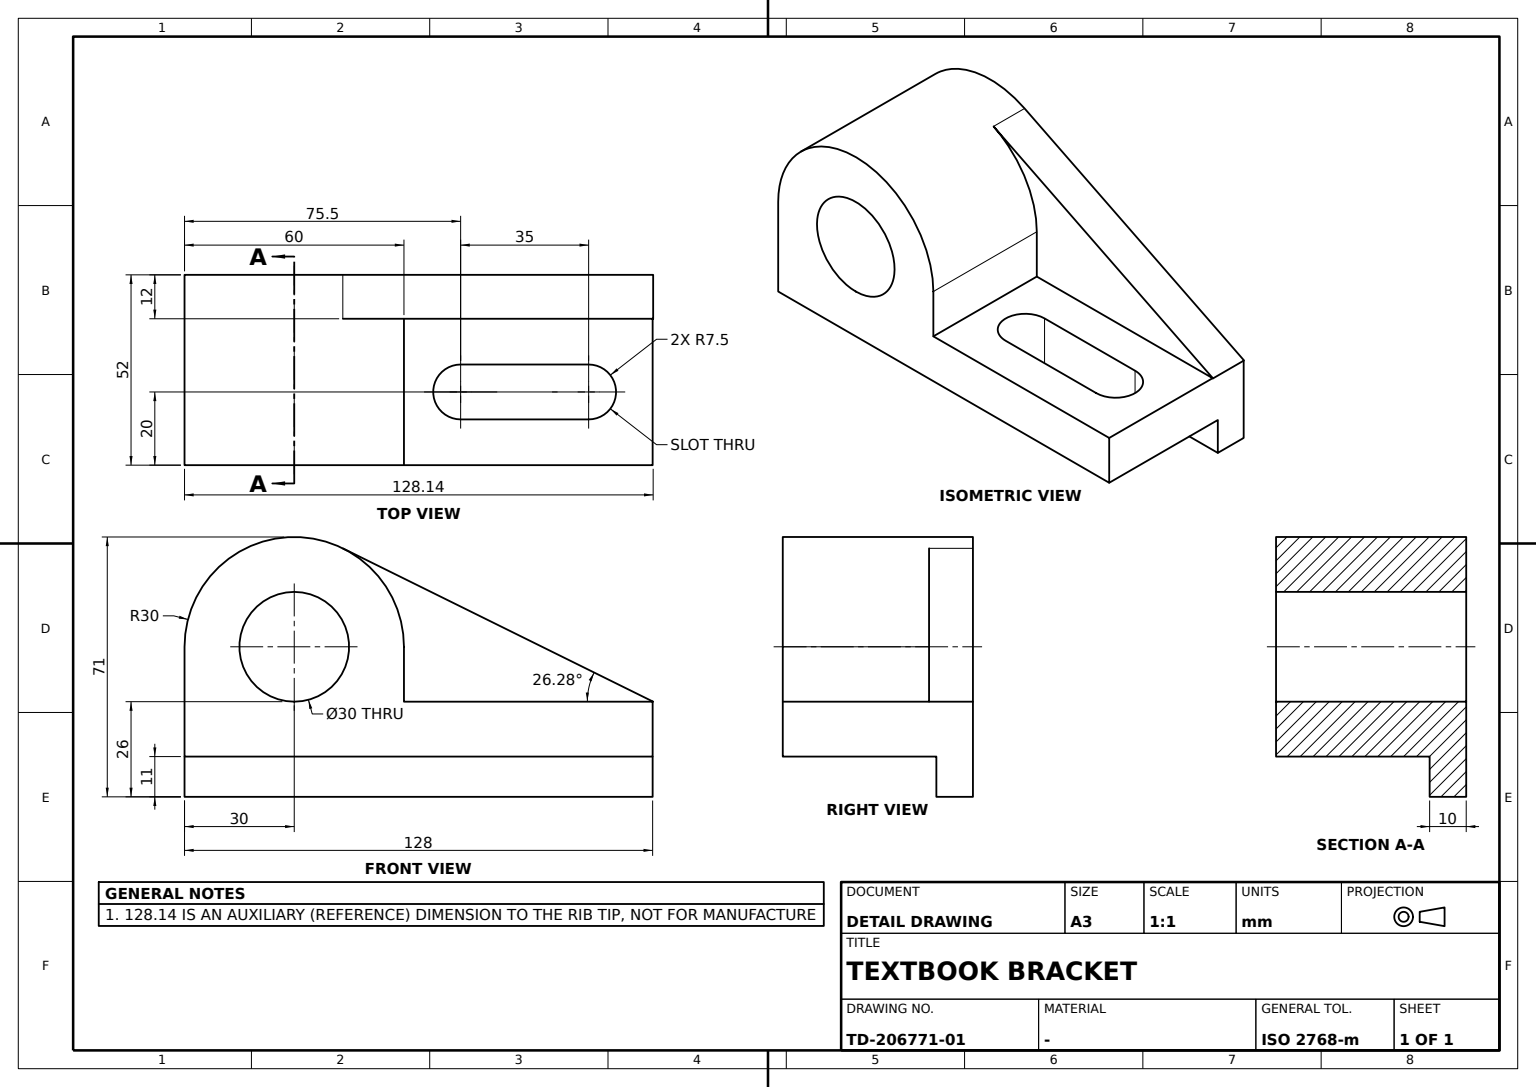
ISO-10303-21;
HEADER;
FILE_DESCRIPTION((''),'2;1');
FILE_NAME('','',(''),(''),'','','');
FILE_SCHEMA(('AUTOMOTIVE_DESIGN'));
ENDSEC;
DATA;
#1=APPLICATION_CONTEXT('');
#2=PRODUCT_CONTEXT('',#1,'mechanical');
#3=PRODUCT('','','',(#2));
#4=PRODUCT_DEFINITION_FORMATION('','',#3);
#5=PRODUCT_DEFINITION_CONTEXT('',#1,'design');
#6=PRODUCT_DEFINITION('','',#4,#5);
#7=PRODUCT_DEFINITION_SHAPE('','',#6);
#8=(LENGTH_UNIT()NAMED_UNIT(*)SI_UNIT(.MILLI.,.METRE.));
#9=(NAMED_UNIT(*)PLANE_ANGLE_UNIT()SI_UNIT($,.RADIAN.));
#10=(NAMED_UNIT(*)SI_UNIT($,.STERADIAN.)SOLID_ANGLE_UNIT());
#11=UNCERTAINTY_MEASURE_WITH_UNIT(LENGTH_MEASURE(0.005),#8,'distance_accuracy_value','');
#12=(GEOMETRIC_REPRESENTATION_CONTEXT(3)GLOBAL_UNCERTAINTY_ASSIGNED_CONTEXT((#11))GLOBAL_UNIT_ASSIGNED_CONTEXT((#8,#9,#10))REPRESENTATION_CONTEXT('',''));
#13=CARTESIAN_POINT('',(26.,-30.,0.));
#14=VERTEX_POINT('',#13);
#15=CARTESIAN_POINT('',(26.,-30.,-30.));
#16=VERTEX_POINT('',#15);
#17=DIRECTION('',(0.,0.,-1.));
#18=VECTOR('',#17,1000.);
#19=LINE('',#13,#18);
#20=EDGE_CURVE('',#14,#16,#19,.T.);
#21=ORIENTED_EDGE('',*,*,#20,.T.);
#22=CARTESIAN_POINT('',(26.,98.,-30.));
#23=VERTEX_POINT('',#22);
#24=CARTESIAN_POINT('',(26.,0.,-30.));
#25=DIRECTION('',(0.,1.,0.));
#26=VECTOR('',#25,1000.);
#27=LINE('',#24,#26);
#28=EDGE_CURVE('',#16,#23,#27,.T.);
#29=ORIENTED_EDGE('',*,*,#28,.T.);
#30=CARTESIAN_POINT('',(26.,98.,-15.));
#31=VERTEX_POINT('',#30);
#32=CARTESIAN_POINT('',(26.,98.,0.));
#33=DIRECTION('',(0.,0.,1.));
#34=VECTOR('',#33,1000.);
#35=LINE('',#32,#34);
#36=EDGE_CURVE('',#23,#31,#35,.T.);
#37=ORIENTED_EDGE('',*,*,#36,.T.);
#38=CARTESIAN_POINT('',(26.,30.,-15.));
#39=VERTEX_POINT('',#38);
#40=CARTESIAN_POINT('',(26.,0.,-15.));
#41=DIRECTION('',(0.,-1.,0.));
#42=VECTOR('',#41,1000.);
#43=LINE('',#40,#42);
#44=EDGE_CURVE('',#31,#39,#43,.T.);
#45=ORIENTED_EDGE('',*,*,#44,.T.);
#46=CARTESIAN_POINT('',(26.,30.,0.));
#47=VERTEX_POINT('',#46);
#48=LINE('',#46,#34);
#49=EDGE_CURVE('',#39,#47,#48,.T.);
#50=ORIENTED_EDGE('',*,*,#49,.T.);
#51=CARTESIAN_POINT('',(26.,0.,0.));
#52=DIRECTION('',(1.,0.,0.));
#53=AXIS2_PLACEMENT_3D('',#51,#52,#17);
#54=CIRCLE('',#53,30.);
#55=EDGE_CURVE('',#47,#14,#54,.T.);
#56=ORIENTED_EDGE('',*,*,#55,.T.);
#57=EDGE_LOOP('',(#21,#29,#37,#45,#50,#56));
#58=FACE_BOUND('',#57,.T.);
#59=VERTEX_POINT('',#40);
#60=CIRCLE('',#53,15.);
#61=EDGE_CURVE('',#59,#59,#60,.T.);
#62=ORIENTED_EDGE('',*,*,#61,.F.);
#63=EDGE_LOOP('',(#62));
#64=FACE_BOUND('',#63,.T.);
#65=AXIS2_PLACEMENT_3D('',#51,#52,#25);
#66=PLANE('',#65);
#67=ADVANCED_FACE('',(#58,#64),#66,.T.);
#68=CARTESIAN_POINT('',(-16.,98.,-41.));
#69=VERTEX_POINT('',#68);
#70=CARTESIAN_POINT('',(-16.,-30.,-41.));
#71=VERTEX_POINT('',#70);
#72=LINE('',#68,#42);
#73=EDGE_CURVE('',#69,#71,#72,.T.);
#74=ORIENTED_EDGE('',*,*,#73,.T.);
#75=CARTESIAN_POINT('',(-26.,-30.,-41.));
#76=VERTEX_POINT('',#75);
#77=CARTESIAN_POINT('',(0.,-30.,-41.));
#78=VECTOR('',#52,1000.);
#79=LINE('',#77,#78);
#80=EDGE_CURVE('',#76,#71,#79,.T.);
#81=ORIENTED_EDGE('',*,*,#80,.F.);
#82=CARTESIAN_POINT('',(-26.,98.,-41.));
#83=VERTEX_POINT('',#82);
#84=LINE('',#82,#42);
#85=EDGE_CURVE('',#83,#76,#84,.T.);
#86=ORIENTED_EDGE('',*,*,#85,.F.);
#87=LINE('',#82,#78);
#88=EDGE_CURVE('',#83,#69,#87,.T.);
#89=ORIENTED_EDGE('',*,*,#88,.T.);
#90=EDGE_LOOP('',(#74,#81,#86,#89));
#91=FACE_BOUND('',#90,.T.);
#92=AXIS2_PLACEMENT_3D('',#82,#17,#52);
#93=PLANE('',#92);
#94=ADVANCED_FACE('',(#91),#93,.T.);
#95=CARTESIAN_POINT('',(-14.,30.,0.));
#96=VERTEX_POINT('',#95);
#97=CARTESIAN_POINT('',(-14.,13.281713,26.899742));
#98=VERTEX_POINT('',#97);
#99=CARTESIAN_POINT('',(-14.,0.,0.));
#100=AXIS2_PLACEMENT_3D('',#99,#52,#17);
#101=CIRCLE('',#100,30.);
#102=EDGE_CURVE('',#96,#98,#101,.T.);
#103=ORIENTED_EDGE('',*,*,#102,.T.);
#104=CARTESIAN_POINT('',(-26.,13.281713,26.899742));
#105=VERTEX_POINT('',#104);
#106=CARTESIAN_POINT('',(0.,13.281713,26.899742));
#107=LINE('',#106,#78);
#108=EDGE_CURVE('',#105,#98,#107,.T.);
#109=ORIENTED_EDGE('',*,*,#108,.F.);
#110=CARTESIAN_POINT('',(-26.,-30.,0.));
#111=VERTEX_POINT('',#110);
#112=CARTESIAN_POINT('',(-26.,0.,0.));
#113=AXIS2_PLACEMENT_3D('',#112,#52,#17);
#114=CIRCLE('',#113,30.);
#115=EDGE_CURVE('',#105,#111,#114,.T.);
#116=ORIENTED_EDGE('',*,*,#115,.T.);
#117=CARTESIAN_POINT('',(0.,-30.,0.));
#118=LINE('',#117,#78);
#119=EDGE_CURVE('',#111,#14,#118,.T.);
#120=ORIENTED_EDGE('',*,*,#119,.T.);
#121=ORIENTED_EDGE('',*,*,#55,.F.);
#122=CARTESIAN_POINT('',(0.,30.,0.));
#123=LINE('',#122,#78);
#124=EDGE_CURVE('',#96,#47,#123,.T.);
#125=ORIENTED_EDGE('',*,*,#124,.F.);
#126=EDGE_LOOP('',(#103,#109,#116,#120,#121,#125));
#127=FACE_BOUND('',#126,.T.);
#128=CARTESIAN_POINT('',(0.,0.,0.));
#129=AXIS2_PLACEMENT_3D('',#128,#52,#25);
#130=CYLINDRICAL_SURFACE('',#129,30.);
#131=ADVANCED_FACE('',(#127),#130,.T.);
#132=CARTESIAN_POINT('',(-1.5,80.5,-15.));
#133=VERTEX_POINT('',#132);
#134=CARTESIAN_POINT('',(-1.5,80.5,-30.));
#135=VERTEX_POINT('',#134);
#136=CARTESIAN_POINT('',(-1.5,80.5,-28.66));
#137=LINE('',#136,#34);
#138=EDGE_CURVE('',#133,#135,#137,.F.);
#139=ORIENTED_EDGE('',*,*,#138,.F.);
#140=CARTESIAN_POINT('',(-1.5,45.5,-15.));
#141=VERTEX_POINT('',#140);
#142=LINE('',#140,#26);
#143=EDGE_CURVE('',#141,#133,#142,.T.);
#144=ORIENTED_EDGE('',*,*,#143,.F.);
#145=CARTESIAN_POINT('',(-1.5,45.5,-30.));
#146=VERTEX_POINT('',#145);
#147=CARTESIAN_POINT('',(-1.5,45.5,-28.66));
#148=LINE('',#147,#34);
#149=EDGE_CURVE('',#141,#146,#148,.F.);
#150=ORIENTED_EDGE('',*,*,#149,.T.);
#151=CARTESIAN_POINT('',(-1.5,-30.,-30.));
#152=LINE('',#151,#26);
#153=EDGE_CURVE('',#146,#135,#152,.T.);
#154=ORIENTED_EDGE('',*,*,#153,.T.);
#155=EDGE_LOOP('',(#139,#144,#150,#154));
#156=FACE_BOUND('',#155,.T.);
#157=DIRECTION('',(-1.,0.,0.));
#158=AXIS2_PLACEMENT_3D('',#140,#157,#25);
#159=PLANE('',#158);
#160=ADVANCED_FACE('',(#156),#159,.F.);
#161=CARTESIAN_POINT('',(-14.,30.,-15.));
#162=VERTEX_POINT('',#161);
#163=CARTESIAN_POINT('',(0.,30.,-15.));
#164=LINE('',#163,#78);
#165=EDGE_CURVE('',#162,#39,#164,.T.);
#166=ORIENTED_EDGE('',*,*,#165,.F.);
#167=LINE('',#95,#34);
#168=EDGE_CURVE('',#162,#96,#167,.T.);
#169=ORIENTED_EDGE('',*,*,#168,.T.);
#170=ORIENTED_EDGE('',*,*,#124,.T.);
#171=ORIENTED_EDGE('',*,*,#49,.F.);
#172=EDGE_LOOP('',(#166,#169,#170,#171));
#173=FACE_BOUND('',#172,.T.);
#174=AXIS2_PLACEMENT_3D('',#163,#25,#33);
#175=PLANE('',#174);
#176=ADVANCED_FACE('',(#173),#175,.T.);
#177=CARTESIAN_POINT('',(13.5,45.5,-30.));
#178=VERTEX_POINT('',#177);
#179=CARTESIAN_POINT('',(6.,45.5,-30.));
#180=AXIS2_PLACEMENT_3D('',#179,#17,#157);
#181=CIRCLE('',#180,7.5);
#182=EDGE_CURVE('',#178,#146,#181,.T.);
#183=ORIENTED_EDGE('',*,*,#182,.T.);
#184=ORIENTED_EDGE('',*,*,#149,.F.);
#185=CARTESIAN_POINT('',(13.5,45.5,-15.));
#186=VERTEX_POINT('',#185);
#187=CARTESIAN_POINT('',(6.,45.5,-15.));
#188=AXIS2_PLACEMENT_3D('',#187,#33,#52);
#189=CIRCLE('',#188,7.5);
#190=EDGE_CURVE('',#141,#186,#189,.T.);
#191=ORIENTED_EDGE('',*,*,#190,.T.);
#192=CARTESIAN_POINT('',(13.5,45.5,-28.66));
#193=LINE('',#192,#34);
#194=EDGE_CURVE('',#186,#178,#193,.F.);
#195=ORIENTED_EDGE('',*,*,#194,.T.);
#196=EDGE_LOOP('',(#183,#184,#191,#195));
#197=FACE_BOUND('',#196,.T.);
#198=CARTESIAN_POINT('',(6.,45.5,-28.66));
#199=AXIS2_PLACEMENT_3D('',#198,#33,#25);
#200=CYLINDRICAL_SURFACE('',#199,7.5);
#201=ADVANCED_FACE('',(#197),#200,.F.);
#202=CARTESIAN_POINT('',(13.5,80.5,-15.));
#203=VERTEX_POINT('',#202);
#204=LINE('',#185,#26);
#205=EDGE_CURVE('',#186,#203,#204,.T.);
#206=ORIENTED_EDGE('',*,*,#205,.T.);
#207=CARTESIAN_POINT('',(13.5,80.5,-30.));
#208=VERTEX_POINT('',#207);
#209=CARTESIAN_POINT('',(13.5,80.5,-28.66));
#210=LINE('',#209,#34);
#211=EDGE_CURVE('',#203,#208,#210,.F.);
#212=ORIENTED_EDGE('',*,*,#211,.T.);
#213=CARTESIAN_POINT('',(13.5,-30.,-30.));
#214=LINE('',#213,#26);
#215=EDGE_CURVE('',#178,#208,#214,.T.);
#216=ORIENTED_EDGE('',*,*,#215,.F.);
#217=ORIENTED_EDGE('',*,*,#194,.F.);
#218=EDGE_LOOP('',(#206,#212,#216,#217));
#219=FACE_BOUND('',#218,.T.);
#220=AXIS2_PLACEMENT_3D('',#185,#157,#25);
#221=PLANE('',#220);
#222=ADVANCED_FACE('',(#219),#221,.T.);
#223=ORIENTED_EDGE('',*,*,#108,.T.);
#224=CARTESIAN_POINT('',(-14.,98.14217,-15.));
#225=VERTEX_POINT('',#224);
#226=DIRECTION('',(0.,0.896658056,-0.442723763));
#227=VECTOR('',#226,1000.);
#228=LINE('',#97,#227);
#229=EDGE_CURVE('',#98,#225,#228,.T.);
#230=ORIENTED_EDGE('',*,*,#229,.T.);
#231=CARTESIAN_POINT('',(-26.,98.14217,-15.));
#232=VERTEX_POINT('',#231);
#233=CARTESIAN_POINT('',(0.,98.14217,-15.));
#234=LINE('',#233,#78);
#235=EDGE_CURVE('',#232,#225,#234,.T.);
#236=ORIENTED_EDGE('',*,*,#235,.F.);
#237=LINE('',#104,#227);
#238=EDGE_CURVE('',#105,#232,#237,.T.);
#239=ORIENTED_EDGE('',*,*,#238,.F.);
#240=EDGE_LOOP('',(#223,#230,#236,#239));
#241=FACE_BOUND('',#240,.T.);
#242=CARTESIAN_POINT('',(-26.,98.,-14.929804));
#243=DIRECTION('',(0.,-0.442723763,-0.896658056));
#244=AXIS2_PLACEMENT_3D('',#242,#243,#226);
#245=PLANE('',#244);
#246=ADVANCED_FACE('',(#241),#245,.F.);
#247=CARTESIAN_POINT('',(-26.,98.,-15.));
#248=VERTEX_POINT('',#247);
#249=CARTESIAN_POINT('',(-14.,98.,-15.));
#250=VERTEX_POINT('',#249);
#251=CARTESIAN_POINT('',(0.,98.,-15.));
#252=LINE('',#251,#78);
#253=EDGE_CURVE('',#248,#250,#252,.T.);
#254=ORIENTED_EDGE('',*,*,#253,.F.);
#255=LINE('',#247,#26);
#256=EDGE_CURVE('',#248,#232,#255,.T.);
#257=ORIENTED_EDGE('',*,*,#256,.T.);
#258=ORIENTED_EDGE('',*,*,#235,.T.);
#259=LINE('',#249,#26);
#260=EDGE_CURVE('',#250,#225,#259,.T.);
#261=ORIENTED_EDGE('',*,*,#260,.F.);
#262=EDGE_LOOP('',(#254,#257,#258,#261));
#263=FACE_BOUND('',#262,.T.);
#264=AXIS2_PLACEMENT_3D('',#251,#33,#41);
#265=PLANE('',#264);
#266=ADVANCED_FACE('',(#263),#265,.F.);
#267=ORIENTED_EDGE('',*,*,#73,.F.);
#268=CARTESIAN_POINT('',(-16.,98.,-30.));
#269=VERTEX_POINT('',#268);
#270=LINE('',#68,#34);
#271=EDGE_CURVE('',#69,#269,#270,.T.);
#272=ORIENTED_EDGE('',*,*,#271,.T.);
#273=CARTESIAN_POINT('',(-16.,-30.,-30.));
#274=VERTEX_POINT('',#273);
#275=LINE('',#273,#42);
#276=EDGE_CURVE('',#269,#274,#275,.T.);
#277=ORIENTED_EDGE('',*,*,#276,.T.);
#278=CARTESIAN_POINT('',(-16.,-30.,0.));
#279=LINE('',#278,#34);
#280=EDGE_CURVE('',#71,#274,#279,.T.);
#281=ORIENTED_EDGE('',*,*,#280,.F.);
#282=EDGE_LOOP('',(#267,#272,#277,#281));
#283=FACE_BOUND('',#282,.T.);
#284=AXIS2_PLACEMENT_3D('',#68,#52,#33);
#285=PLANE('',#284);
#286=ADVANCED_FACE('',(#283),#285,.T.);
#287=ORIENTED_EDGE('',*,*,#119,.F.);
#288=LINE('',#110,#18);
#289=EDGE_CURVE('',#111,#76,#288,.T.);
#290=ORIENTED_EDGE('',*,*,#289,.T.);
#291=ORIENTED_EDGE('',*,*,#80,.T.);
#292=ORIENTED_EDGE('',*,*,#280,.T.);
#293=CARTESIAN_POINT('',(0.,-30.,-30.));
#294=LINE('',#293,#78);
#295=EDGE_CURVE('',#274,#16,#294,.T.);
#296=ORIENTED_EDGE('',*,*,#295,.T.);
#297=ORIENTED_EDGE('',*,*,#20,.F.);
#298=EDGE_LOOP('',(#287,#290,#291,#292,#296,#297));
#299=FACE_BOUND('',#298,.T.);
#300=AXIS2_PLACEMENT_3D('',#117,#41,#17);
#301=PLANE('',#300);
#302=ADVANCED_FACE('',(#299),#301,.T.);
#303=CARTESIAN_POINT('',(-14.,0.,-15.));
#304=LINE('',#303,#42);
#305=EDGE_CURVE('',#250,#162,#304,.T.);
#306=ORIENTED_EDGE('',*,*,#305,.T.);
#307=ORIENTED_EDGE('',*,*,#165,.T.);
#308=ORIENTED_EDGE('',*,*,#44,.F.);
#309=EDGE_CURVE('',#250,#31,#252,.T.);
#310=ORIENTED_EDGE('',*,*,#309,.F.);
#311=EDGE_LOOP('',(#306,#307,#308,#310));
#312=FACE_BOUND('',#311,.T.);
#313=ORIENTED_EDGE('',*,*,#190,.F.);
#314=ORIENTED_EDGE('',*,*,#143,.T.);
#315=CARTESIAN_POINT('',(6.,80.5,-15.));
#316=AXIS2_PLACEMENT_3D('',#315,#33,#52);
#317=CIRCLE('',#316,7.5);
#318=EDGE_CURVE('',#203,#133,#317,.T.);
#319=ORIENTED_EDGE('',*,*,#318,.F.);
#320=ORIENTED_EDGE('',*,*,#205,.F.);
#321=EDGE_LOOP('',(#313,#314,#319,#320));
#322=FACE_BOUND('',#321,.T.);
#323=ADVANCED_FACE('',(#312,#322),#265,.T.);
#324=ORIENTED_EDGE('',*,*,#28,.F.);
#325=ORIENTED_EDGE('',*,*,#295,.F.);
#326=ORIENTED_EDGE('',*,*,#276,.F.);
#327=CARTESIAN_POINT('',(0.,98.,-30.));
#328=LINE('',#327,#78);
#329=EDGE_CURVE('',#269,#23,#328,.T.);
#330=ORIENTED_EDGE('',*,*,#329,.T.);
#331=EDGE_LOOP('',(#324,#325,#326,#330));
#332=FACE_BOUND('',#331,.T.);
#333=CARTESIAN_POINT('',(6.,80.5,-30.));
#334=AXIS2_PLACEMENT_3D('',#333,#17,#157);
#335=CIRCLE('',#334,7.5);
#336=EDGE_CURVE('',#135,#208,#335,.T.);
#337=ORIENTED_EDGE('',*,*,#336,.F.);
#338=ORIENTED_EDGE('',*,*,#153,.F.);
#339=ORIENTED_EDGE('',*,*,#182,.F.);
#340=ORIENTED_EDGE('',*,*,#215,.T.);
#341=EDGE_LOOP('',(#337,#338,#339,#340));
#342=FACE_BOUND('',#341,.T.);
#343=AXIS2_PLACEMENT_3D('',#293,#17,#25);
#344=PLANE('',#343);
#345=ADVANCED_FACE('',(#332,#342),#344,.T.);
#346=CARTESIAN_POINT('',(-26.,0.,-15.));
#347=VERTEX_POINT('',#346);
#348=CIRCLE('',#113,15.);
#349=EDGE_CURVE('',#347,#347,#348,.T.);
#350=ORIENTED_EDGE('',*,*,#349,.T.);
#351=EDGE_LOOP('',(#350));
#352=FACE_BOUND('',#351,.T.);
#353=ORIENTED_EDGE('',*,*,#289,.F.);
#354=ORIENTED_EDGE('',*,*,#115,.F.);
#355=ORIENTED_EDGE('',*,*,#238,.T.);
#356=ORIENTED_EDGE('',*,*,#256,.F.);
#357=CARTESIAN_POINT('',(-26.,98.,0.));
#358=LINE('',#357,#34);
#359=EDGE_CURVE('',#83,#248,#358,.T.);
#360=ORIENTED_EDGE('',*,*,#359,.F.);
#361=ORIENTED_EDGE('',*,*,#85,.T.);
#362=EDGE_LOOP('',(#353,#354,#355,#356,#360,#361));
#363=FACE_BOUND('',#362,.T.);
#364=AXIS2_PLACEMENT_3D('',#112,#52,#25);
#365=PLANE('',#364);
#366=ADVANCED_FACE('',(#352,#363),#365,.F.);
#367=ORIENTED_EDGE('',*,*,#88,.F.);
#368=ORIENTED_EDGE('',*,*,#359,.T.);
#369=ORIENTED_EDGE('',*,*,#253,.T.);
#370=ORIENTED_EDGE('',*,*,#309,.T.);
#371=ORIENTED_EDGE('',*,*,#36,.F.);
#372=ORIENTED_EDGE('',*,*,#329,.F.);
#373=ORIENTED_EDGE('',*,*,#271,.F.);
#374=EDGE_LOOP('',(#367,#368,#369,#370,#371,#372,#373));
#375=FACE_BOUND('',#374,.T.);
#376=AXIS2_PLACEMENT_3D('',#327,#25,#33);
#377=PLANE('',#376);
#378=ADVANCED_FACE('',(#375),#377,.T.);
#379=ORIENTED_EDGE('',*,*,#138,.T.);
#380=ORIENTED_EDGE('',*,*,#336,.T.);
#381=ORIENTED_EDGE('',*,*,#211,.F.);
#382=ORIENTED_EDGE('',*,*,#318,.T.);
#383=EDGE_LOOP('',(#379,#380,#381,#382));
#384=FACE_BOUND('',#383,.T.);
#385=CARTESIAN_POINT('',(6.,80.5,-28.66));
#386=AXIS2_PLACEMENT_3D('',#385,#33,#25);
#387=CYLINDRICAL_SURFACE('',#386,7.5);
#388=ADVANCED_FACE('',(#384),#387,.F.);
#389=ORIENTED_EDGE('',*,*,#229,.F.);
#390=ORIENTED_EDGE('',*,*,#102,.F.);
#391=ORIENTED_EDGE('',*,*,#168,.F.);
#392=ORIENTED_EDGE('',*,*,#305,.F.);
#393=ORIENTED_EDGE('',*,*,#260,.T.);
#394=EDGE_LOOP('',(#389,#390,#391,#392,#393));
#395=FACE_BOUND('',#394,.T.);
#396=AXIS2_PLACEMENT_3D('',#99,#52,#25);
#397=PLANE('',#396);
#398=ADVANCED_FACE('',(#395),#397,.T.);
#399=ORIENTED_EDGE('',*,*,#61,.T.);
#400=EDGE_LOOP('',(#399));
#401=FACE_BOUND('',#400,.T.);
#402=ORIENTED_EDGE('',*,*,#349,.F.);
#403=EDGE_LOOP('',(#402));
#404=FACE_BOUND('',#403,.T.);
#405=CYLINDRICAL_SURFACE('',#129,15.);
#406=ADVANCED_FACE('',(#401,#404),#405,.F.);
#407=CLOSED_SHELL('',(#67,#94,#131,#160,#176,#201,#222,#246,#266,#286,#302,#323,#345,#366,#378,#388,#398,#406));
#408=MANIFOLD_SOLID_BREP('',#407);
#409=ADVANCED_BREP_SHAPE_REPRESENTATION('',(#408),#12);
#410=SHAPE_DEFINITION_REPRESENTATION(#7,#409);
ENDSEC;
END-ISO-10303-21;
